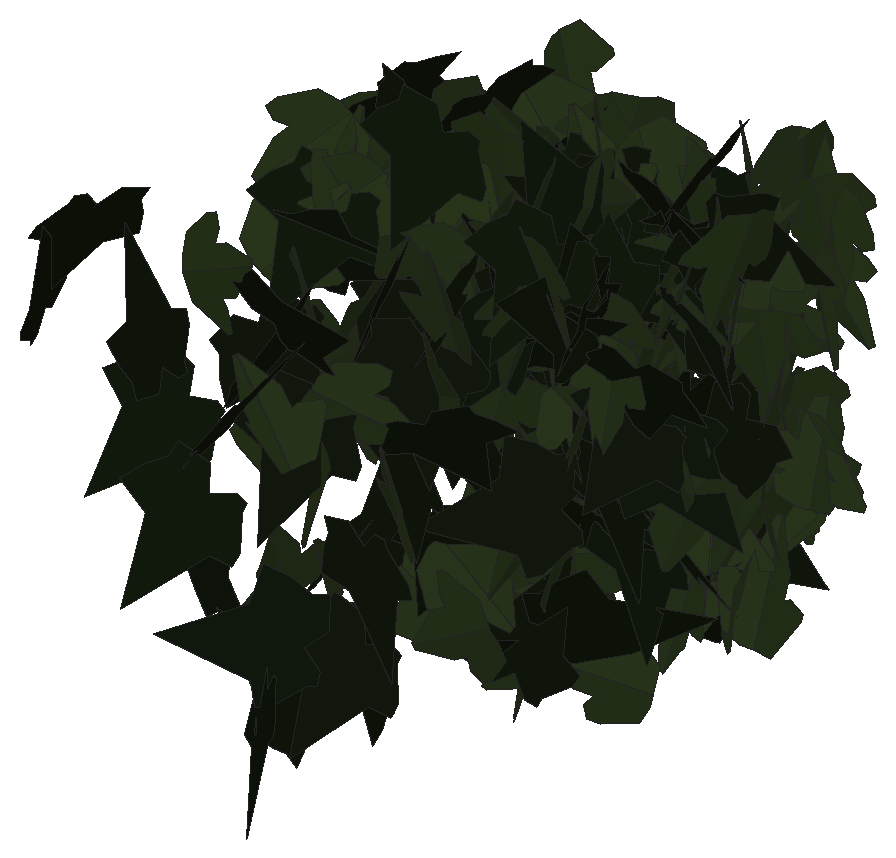
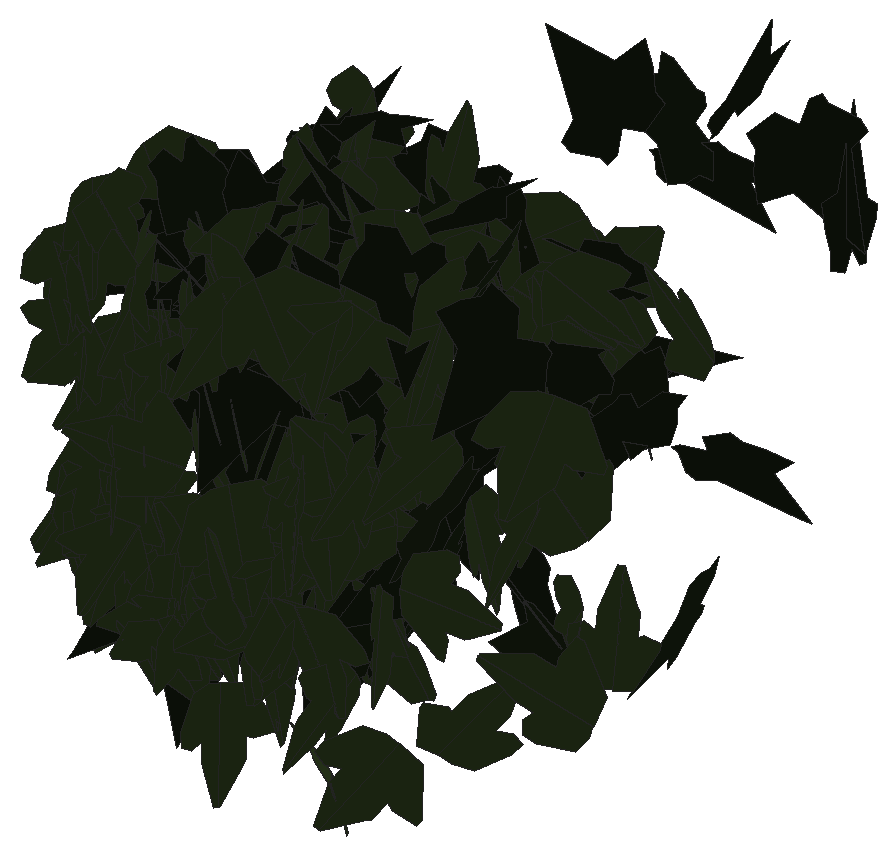
# SketchUp Ruby script. Lengths in inches.
U = 1.inch
M = Sketchup.active_model
def pt(a) = Geom::Point3d.new(a.map { |v| v * U })
def face(e, loops, mat)
  f = e.add_face(loops[0].map { |a| pt(a) })
  loops[1..].each { |l| e.add_face(l.map { |a| pt(a) }).erase! }
  f.material = f.back_material = mat if mat
  f
end
# faces: each face lists its corners as indices into pts; further lists are holes
def faces(e, pts, list, mat = nil) = list.each { |f| face(e, (f[0].is_a?(Array) ? f : [f]).map { |l| l.map { |i| pts[i] } }, mat) }
# xy, xz, yz: faces in a plane at the given z, y or x. An outline is a flat list of corners, or four numbers for a rectangle; further outlines are holes
def ring(l) = l.size == 4 ? [[l[0], l[1]], [l[2], l[1]], [l[2], l[3]], [l[0], l[3]]] : l.each_slice(2).to_a
def flat(e, list, mat, &to3) = list.each { |f| face(e, (f[0].is_a?(Array) ? f : [f]).map { |l| ring(l).map { |u, v| to3.(u, v) } }, mat) }
def xy(e, z, list, mat = nil) = flat(e, list, mat) { |x, y| [x, y, z] }
def xz(e, y, list, mat = nil) = flat(e, list, mat) { |x, z| [x, y, z] }
def yz(e, x, list, mat = nil) = flat(e, list, mat) { |y, z| [x, y, z] }
def lines(e, pts, list) = list.each { |a, b| e.add_line(pt(pts[a]), pt(pts[b])) }
# prism: a flat outline (further loops are holes) pulled along v
def prism(e, loops, v, mat = nil)
  f = face(e, loops, mat); d = Geom::Vector3d.new(v.map { |x| x * U })
  f.pushpull(f.normal.samedirection?(d) ? d.length : -d.length)
end
def box(e, o, s, mat = nil) = prism(e, [[o, [o[0] + s[0], o[1], o[2]], [o[0] + s[0], o[1] + s[1], o[2]], [o[0], o[1] + s[1], o[2]]]], [0, 0, s[2]], mat)
def at(x, y, z, deg = 0) = Geom::Transformation.translation(pt([x, y, z])) * Geom::Transformation.rotation(ORIGIN, Z_AXIS, deg.degrees)
def axes(o, x, y, z) = Geom::Transformation.new([*x, 0, *y, 0, *z, 0, *pt(o).to_a, 1])
def part(name) = M.definitions.add(name)
# library, detail: a bought-in or finely detailed component or shape, given as its bounding box
def library(name, o, s) = part(name).tap { |d| box(d.entities, o, s) }
def detail(e, o, s) = box(e.add_group.entities, o, s)
def put(e, d, t, mat = nil) = e.add_instance(d, t).tap { |i| i.material = mat if mat }
def group(e, t, mat = nil) = e.add_group.tap { |g| g.transformation = t; g.material = mat if mat }.entities
root = M.entities
M.materials.add("efeu1").color = [18, 25, 13]
M.materials.add("efeu2").color = [43, 57, 29]
c1 = part("ivyleaf_10")
p = [[0,0.5,-0.03],[-0.0625,2.02,-0.43],[-0.19,2.01,-0.46],[-0.54,1.05,-0.29],[-0.52,0.625,-0.18],[-0.83,0.76,-0.28],
  [-1.16,0.64,-0.33],[-1.15,0.33,-0.24],[-0.77,-0.39,0.02],[-0.3,-0.51,0.16],[0.04,-0.48,0.23],[-0.02,2.01,-0.4375],
  [-0.06,2.01,-0.43],[0.04,-0.49,0.23],[0.67,-0.49,0.14],[1.38,0.36,-0.2],[1.375,0.51,-0.24],[0.81,0.65,-0.19],
  [0.62,0.59,-0.15],[0.6,1.09,-0.28],[0.5,1.23,-0.31]]
faces(c1.entities,p,[[0,1,2,3,4,5,6,7,8,9,10],[11,12,0,13,14,15,16,17,18,19,20]],"efeu2")
c2 = part("ivyleaf_9")
p = [[1.54,2.16,1.25],[1.36,2.04,1.19],[-0.21,0.99,0.68],[-0.71,1.11,0.82],[-0.85,0.86,0.67],[-0.8,0.17,0.21],
  [-0.9,-0.01,0.1],[-0.67,-0.16,-0.02],[-0.08,-0.08,-0.05],[-0.03,-0.6,-0.4],[0.65,-0.88,-0.66],[0.83,-0.6,-0.49],
  [1.29,-0.42,-0.43],[1.8125,-0.07,-0.26],[1.21,0.44,0.15]]
faces(c2.entities,p,[[0,1,2,3,4,5,6,7,8,9,10,11,12,13,14]],"efeu1")
put(root,c1,axes([4.1875,224.93,203.2],[-0.1697,-0.07325,0.46458],[0.41933,0.2001,0.18472],[-0.21299,0.45232,-0.00648]))
put(root,c2,axes([4.59,220.26,206.02],[0.03494,0.24772,0.37035],[-0.11703,-0.34116,0.25706],[0.45365,-0.10709,0.03779]))
put(root,c1,axes([4.64,224.79,206.06],[-0.40343,-0.25391,-0.15091],[0.12885,0.07858,-0.47668],[0.26579,-0.4235,0.00203]))
put(root,c2,axes([4.91,221.93,204.38],[-0.43733,-0.15279,0.04548],[-0.04405,-0.01579,-0.45011],[0.16589,-0.40698,0.00039]))
put(root,c2,axes([5.05,220.43,207.12],[-0.05074,0.32429,-0.29754],[0.02517,-0.28547,-0.3405],[-0.46637,-0.05069,0.01399]))
put(root,c1,axes([5.375,223.53,206.75],[0.32878,0.07304,-0.3141],[-0.31526,-0.07769,-0.32554],[-0.11502,0.42173,-0.00557]))
put(root,c2,axes([5.04,222.01,202.73],[0.33996,-0.26991,-0.13674],[-0.10665,0.08682,-0.43124],[0.30621,0.3299,0.00162]))
put(root,c1,axes([4.91,222.18,205.66],[0.17929,-0.09629,-0.40599],[0.35577,-0.20958,0.19946],[-0.24898,-0.36882,-0.00735]))
put(root,c2,axes([5.21,224.53,206.61],[0.21832,0.33606,0.19573],[0.10391,0.16176,-0.40786],[-0.4028,0.22388,0.00088]))
put(root,c1,axes([5.71,225.24,204.04],[0.01886,0.02284,-0.45141],[-0.45168,0.11918,-0.01097],[0.12784,0.41773,0.02782]))
put(root,c2,axes([5.29,222.61,204.98],[0.08106,-0.27792,-0.33917],[-0.05368,0.3232,-0.29834],[0.45963,0.08676,0.02497]))
put(root,c1,axes([5.51,222.69,202.25],[-0.12317,-0.38419,-0.17594],[-0.02837,-0.16843,0.41622],[-0.45248,0.11514,0.0218]))
put(root,c1,axes([5.39,222.75,205.75],[0.27183,0.16125,-0.32867],[0.29159,0.16433,0.31083],[0.24859,-0.36908,-0.0052]))
put(root,c1,axes([5.71,223.23,206.21],[0.01419,0.31497,-0.31174],[0.01599,0.29939,0.32785],[0.46931,-0.01972,-0.00174]))
put(root,c2,axes([5.73,223.18,206.26],[-0.31837,-0.3187,0.02862],[-0.02124,-0.01929,-0.45149],[0.34482,-0.29544,-0.00139]))
put(root,c1,axes([5.59,223.17,203.97],[-0.15528,-0.36601,0.19342],[0.07202,0.17362,0.40897],[-0.43751,0.15849,-0.00133]))
put(root,c2,axes([5.71,223.18,202.38],[-0.22203,0.36028,-0.13624],[-0.07015,0.11376,0.4314],[0.40804,0.2156,0.00003]))
put(root,c2,axes([5.54,222.15,204.72],[0.09632,0.39174,0.17344],[-0.04238,-0.16211,0.41783],[0.45786,-0.09741,0.00218]))
put(root,c1,axes([5.89,223.38,206.35],[0.26009,0.1336,-0.35019],[-0.32984,-0.14257,-0.286],[-0.21041,0.38865,0.01546]))
put(root,c1,axes([5.77,222.7,205.28],[-0.35795,0.25236,0.13029],[0.09959,-0.08561,0.43306],[0.28752,0.34382,0.0122]))
put(root,c1,axes([5.85,223.49,204.02],[-0.06806,0.27457,0.34471],[-0.11059,0.31581,-0.29232],[-0.4515,-0.11874,0.01964]))
put(root,c1,axes([5.75,225.01,205.41],[0.04742,0.23194,0.37999],[0.05868,0.36139,-0.24538],[-0.4637,0.06945,0.00781]))
put(root,c2,axes([5.48,223.01,205.72],[0.29751,-0.01523,0.34976],[0.36233,-0.02377,-0.28691],[0.03028,0.43408,-0.00344]))
put(root,c1,axes([5.85,223.35,204.84],[0.08243,-0.36347,0.23552],[-0.01128,0.22839,0.38488],[-0.46237,-0.07037,0.03259]))
put(root,c1,axes([6.08,224.6875,206.58],[0.04798,0.09131,-0.48924],[-0.18918,-0.45127,-0.10278],[-0.46034,0.19497,-0.00875]))
put(root,c1,axes([6.05,224.69,206.42],[-0.44092,0.23576,-0.00349],[0.00297,-0.00185,-0.49999],[-0.23576,-0.44093,0.00023]))
put(root,c1,axes([5.91,225.62,202.35],[-0.365,-0.11682,-0.25762],[0.25231,0.08236,-0.37188],[0.15436,-0.41085,-0.0013]))
put(root,c1,axes([5.95,222.74,202.62],[-0.24505,0.2853,-0.24686],[0.15233,-0.19105,-0.37904],[-0.37075,-0.26707,0.00743]))
put(root,c2,axes([5.875,224.19,206.8],[0.11049,-0.37667,0.19972],[0.05839,-0.18431,-0.40591],[0.45287,0.11566,0.0036]))
put(root,c1,axes([6.16,223.84,204.05],[0.11861,-0.42089,0.00439],[0.00599,-0.00292,-0.45235],[0.45454,0.10986,0.00482]))
put(root,c2,axes([6.04,223.84,205.23],[0.01774,-0.29834,-0.32879],[-0.02163,0.31552,-0.31073],[0.46897,0.02584,-0.00189]))
put(root,c1,axes([6.3,224.01,201.72],[0.18967,0.31034,0.25911],[-0.13634,-0.21482,0.37083],[0.40762,-0.21625,0.00347]))
put(root,c1,axes([6.21,224.6,205.5],[-0.08774,-0.27767,-0.33784],[0.12661,0.30349,-0.30029],[0.44383,-0.14147,0.01888]))
put(root,c1,axes([6.28,225.4,205.21],[0.02776,-0.11632,-0.48549],[0.02716,0.48587,-0.11486],[0.49849,-0.01999,0.0333]))
put(root,c2,axes([6.41,222.98,202.81],[-0.3971,0.21835,-0.08288],[-0.08135,0.02916,0.44453],[0.23749,0.37509,0.01369]))
put(root,c2,axes([6.45,224.51,207.04],[0.05714,0.43158,-0.01349],[-0.00179,-0.01287,-0.4522],[-0.46631,0.05293,0.00008]))
put(root,c1,axes([6.34,225.85,206.84],[-0.01928,0.43461,-0.00484],[0.00288,-0.00455,-0.45237],[-0.4694,-0.01787,-0.00257]))
put(root,c2,axes([6.11,224.52,204.37],[0.21804,-0.41741,0.16801],[0.09712,-0.13864,-0.47048],[0.43935,0.2378,0.02062]))
put(root,c2,axes([6.09,224.21,206.42],[0.28246,-0.36735,0.18779],[0.11329,-0.14977,-0.46339],[0.39671,0.30433,-0.00137]))
put(root,c2,axes([6.3125,224.04,203.78],[0.32495,-0.22821,-0.22454],[-0.18254,0.13441,-0.39272],[0.286,0.34508,0.00447]))
put(root,c2,axes([6.57,219.5,206.44],[-0.12179,-0.33455,0.26431],[0.08473,0.24174,0.36715],[-0.44576,0.13736,-0.00242]))
put(root,c1,axes([6.63,224.68,203.27],[0.06532,-0.31686,-0.3035],[-0.05497,0.28737,-0.33547],[0.46198,0.07899,0.00299]))
put(root,c1,axes([6.75,225.37,201.76],[0.28586,-0.01067,0.35884],[-0.30725,0.23953,0.23467],[-0.21117,-0.36295,0.14432]))
put(root,c1,axes([6.65,223.71,206.62],[0.30392,0.25824,-0.21653],[-0.17165,-0.13468,-0.39715],[-0.31446,0.3231,0.00751]))
put(root,c1,axes([6.95,224.8,206.32],[-0.32488,0.05136,-0.32239],[-0.3354,0.01678,0.3163],[0.05169,0.43163,0.02607]))
put(root,c1,axes([6.45,225.2,206.56],[0.33672,0.25277,0.26969],[0.21818,0.15857,-0.42102],[-0.29836,0.40121,-0.00351]))
put(root,c1,axes([6.77,224.46,206.58],[-0.36671,-0.27159,0.01364],[-0.01095,-0.00833,-0.45219],[0.29345,-0.3397,0.00018]))
put(root,c1,axes([6.76,224.07,205.87],[-0.10194,-0.42462,0.00382],[-0.0007,-0.00362,-0.45238],[0.45861,-0.09439,0.00016]))
put(root,c2,axes([6.65,223.58,207.07],[-0.18972,-0.37844,0.12799],[0.01636,-0.14079,-0.42776],[0.42948,-0.16182,0.07283]))
put(root,c2,axes([6.4375,224.2,203.67],[0.45219,-0.10966,0.04531],[0.0455,-0.0111,-0.45013],[0.11904,0.42081,-0.00006]))
put(root,c1,axes([6.49,224.41,202.5],[0.36899,-0.14762,-0.23419],[0.22216,-0.09164,0.38706],[-0.18763,-0.39879,-0.00225]))
put(root,c1,axes([6.74,224.65,206.29],[-0.3796,-0.23626,-0.1033],[0.08975,0.05442,-0.44045],[0.26184,-0.36117,0.00121]))
put(root,c1,axes([6.92,225.6875,204.99],[-0.35044,0.24683,0.25743],[-0.22486,0.12722,-0.42808],[-0.27682,-0.4158,0.02184]))
put(root,c2,axes([6.86,224.59,206.06],[0.03769,0.43317,0.01992],[0.01042,0.01844,-0.45188],[-0.46817,0.03528,-0.00846]))
put(root,c1,axes([6.74,225.22,202.62],[-0.0201,0.24666,0.37214],[-0.05921,0.35396,-0.25672],[-0.46562,-0.05566,0.01658]))
put(root,c1,axes([6.79,224.74,205.96],[0.19796,0.35466,-0.17965],[-0.11675,-0.13803,-0.41403],[-0.40975,0.21068,0.03117]))
put(root,c1,axes([6.6875,224.875,205.64],[-0.34617,-0.21219,-0.21177],[0.20034,0.08785,-0.39887],[0.24647,-0.36943,0.02679]))
put(root,c1,axes([6.6875,225.25,205.1],[0.17132,0.27764,-0.30672],[0.15529,0.2575,0.33254],[0.40896,-0.21409,0.00222]))
put(root,c1,axes([6.9,225.24,204.6],[-0.36722,-0.26745,0.04743],[-0.04215,-0.02416,-0.44987],[0.28997,-0.34221,-0.00531]))
put(root,c2,axes([7.1,224.42,204.9],[-0.28827,-0.08559,0.34595],[-0.34028,-0.10674,-0.29149],[0.14771,-0.41292,0.00364]))
put(root,c1,axes([6.97,220.81,205.1],[0.37699,0.06883,0.2603],[-0.26494,-0.04966,0.37001],[0.09165,-0.42664,-0.00108]))
put(root,c1,axes([6.71,225.3,204.78],[0.40688,0.17958,-0.12757],[0.1197,0.05255,0.43404],[0.20208,-0.3927,-0.00025]))
put(root,c1,axes([6.53,225.01,204.43],[-0.02062,-0.00386,-0.45195],[0.46593,0.05222,-0.0202],[0.05653,-0.43184,0.0016]))
put(root,c1,axes([6.89,225.49,203.4],[0.49225,-0.03479,-0.08051],[-0.08032,0.00552,-0.49348],[0.03523,0.49876,-0.00016]))
put(root,c2,axes([7.18,221.91,202.37],[0.01916,0.01196,-0.45185],[-0.46822,-0.03043,-0.01928],[-0.03338,0.43377,0.01111]))
put(root,c1,axes([7.04,224.07,206.87],[-0.4832,-0.0062,0.12836],[-0.12806,-0.01896,-0.48295],[0.01085,-0.4996,0.01674]))
put(root,c1,axes([7.1,224.8125,204.15],[-0.14457,-0.02266,0.4298],[-0.16943,-0.39916,-0.07561],[0.41365,-0.17142,0.11925]))
put(root,c2,axes([6.75,224.66,206.04],[0.19302,0.39535,0.03259],[-0.02879,-0.02232,0.45095],[0.42735,-0.18007,0.01566]))
put(root,c2,axes([6.75,224.58,205.84],[0.30492,0.04251,0.34132],[0.26166,0.2673,-0.25277],[-0.24345,0.34054,0.15581]))
put(root,c1,axes([7.07,225.18,204.66],[0.27383,0.28604,-0.21596],[-0.16674,-0.14026,-0.397],[-0.3434,0.2962,0.02056]))
put(root,c2,axes([7.0625,222.37,206.32],[-0.26031,0.19627,-0.31649],[0.25558,-0.19134,-0.32326],[-0.29603,-0.33778,-0.00079]))
put(root,c1,axes([6.95,224.34,206.0625],[0.03067,-0.14695,-0.42478],[0.06462,-0.40408,0.15552],[-0.46432,-0.06595,-0.00642]))
put(root,c1,axes([7.12,225.27,204.12],[0.13945,0.24481,-0.34902],[-0.15471,-0.30363,-0.28767],[-0.42111,0.19262,-0.00989]))
put(root,c2,axes([6.75,224.11,205.75],[0.20544,-0.18803,-0.35677],[0.40603,-0.0176,0.22684],[-0.11681,-0.39187,0.16101]))
put(root,c2,axes([7.16,221.07,205.34],[-0.39959,-0.20611,-0.10319],[0.0935,0.04848,-0.44047],[0.22868,-0.37999,-0.00022]))
put(root,c1,axes([7.02,222.82,206.36],[-0.39804,-0.11368,-0.20922],[0.2037,0.07079,-0.40096],[0.14417,-0.41387,-0.01112]))
put(root,c2,axes([6.72,224.38,205.27],[0.33615,0.08318,-0.36067],[0.34408,0.10935,0.3459],[0.13642,-0.48075,0.01628]))
put(root,c1,axes([7.14,223.74,205.23],[-0.07646,-0.39956,-0.16301],[0.10948,0.1388,-0.41559],[0.45042,-0.10156,0.07335]))
put(root,c1,axes([7.08,224.91,204.2],[-0.27523,-0.28491,-0.21592],[0.21066,0.09944,-0.39092],[0.31715,-0.31331,0.07228]))
put(root,c2,axes([7.02,224.38,205.26],[0.14069,-0.4475,-0.17306],[-0.04406,0.16753,-0.46903],[0.47777,0.14723,0.0077]))
put(root,c1,axes([7.15,225.32,203.26],[-0.06355,0.41424,-0.12379],[0.02021,-0.11757,-0.43513],[-0.46504,-0.06171,-0.00199]))
put(root,c1,axes([7.36,223.66,204.5625],[-0.34583,-0.25925,0.14514],[-0.10732,-0.09892,-0.42825],[0.29932,-0.33501,0.01414]))
put(root,c1,axes([7.37,225.54,206.68],[-0.21891,-0.41701,0.16787],[-0.05523,-0.16035,-0.47036],[0.44613,-0.22448,0.02415]))
put(root,c2,axes([7.39,219.14,205.43],[-0.42486,-0.18545,-0.00949],[0.00857,0.00458,-0.4523],[0.20034,-0.39346,-0.00079]))
put(root,c2,axes([7.14,224.39,204.49],[-0.03088,-0.37745,-0.22291],[0.04429,0.21149,-0.39303],[0.46669,-0.04504,0.02255]))
put(root,c1,axes([7.27,225.47,203.29],[-0.35355,-0.27119,-0.09599],[0.1514,-0.02942,-0.42717],[0.26981,-0.33885,0.11391]))
put(root,c2,axes([7.66,223.83,203.21],[-0.42781,-0.00958,0.18668],[-0.19381,-0.00408,-0.41209],[0.01124,-0.43488,-0.00025]))
put(root,c2,axes([7.29,219.28,205.92],[-0.09415,0.40895,-0.12474],[-0.02748,0.11721,0.43486],[0.45945,0.09082,0.00045]))
put(root,c1,axes([7.17,224.49,204.6],[0.29831,-0.21627,0.33799],[0.27285,-0.19947,-0.36846],[0.29421,0.40428,-0.00099]))
put(root,c2,axes([7.51,220.33,202.65],[0.00879,-0.42348,0.10308],[0.0016,0.09916,0.44049],[-0.46972,-0.00758,0.00343]))
put(root,c1,axes([7.34,225.39,203.78],[0.24286,0.36958,-0.04731],[-0.04172,-0.0297,-0.44955],[-0.39999,0.22749,0.01817]))
put(root,c2,axes([7.09,224.6,202.4],[0.1331,-0.26789,0.40065],[0.15376,-0.37033,-0.29869],[0.45677,0.20272,-0.0162]))
put(root,c1,axes([7.47,220.75,204.91],[0.24236,-0.35034,-0.13208],[-0.06309,0.11334,-0.43253],[0.39748,0.23161,0.01188]))
put(root,c2,axes([7.76,220.0625,203.56],[-0.23864,-0.04809,0.38646],[-0.39428,-0.06951,-0.23512],[0.09112,-0.42671,-0.00525]))
put(root,c1,axes([7.68,225.17,203.84],[-0.1435,-0.09106,0.47023],[-0.23369,-0.41518,-0.15171],[0.41809,-0.26331,0.0766]))
put(root,c2,axes([7.11,220.58,206.55],[0.04935,-0.16782,0.41466],[0.34583,-0.25645,-0.15042],[0.31413,0.3087,0.10046]))
put(root,c1,axes([7.46,224.32,203.82],[-0.16746,-0.39234,-0.11031],[0.07573,0.086,-0.43743],[0.43236,-0.16702,0.0339]))
put(root,c1,axes([7.54,225.23,202.8125],[0.04902,-0.43069,-0.04247],[-0.00393,0.04068,-0.4504],[0.46722,0.04553,0.00067]))
put(root,c1,axes([7.66,225.66,204.41],[-0.3214,-0.37286,0.08762],[-0.05151,-0.07127,-0.49221],[0.37954,-0.32541,0.0074]))
put(root,c1,axes([7.63,225.86,202.42],[-0.13847,-0.40686,-0.08857],[0.01084,0.08607,-0.44333],[0.4488,-0.12761,-0.01662]))
put(root,c1,axes([7.33,221.14,205.59],[-0.21204,-0.09863,-0.39045],[0.38042,0.13152,-0.22751],[0.17616,-0.40274,0.02133]))
put(root,c2,axes([7.75,222.47,206.22],[-0.34524,0.24405,-0.1724],[0.12809,-0.11749,-0.41776],[-0.29175,-0.34038,0.02059]))
put(root,c2,axes([7.75,222.59,203.74],[0.1046,0.30543,-0.30598],[-0.09001,-0.28219,-0.3332],[-0.44908,0.1277,-0.00448]))
put(root,c1,axes([7.54,224.45,203.72],[-0.41875,-0.23529,0.13887],[0.1232,0.06423,0.48031],[-0.24386,0.43648,0.00418]))
put(root,c1,axes([7.57,225.75,203.47],[0.16823,-0.40079,0.06846],[-0.02313,0.0623,0.44718],[-0.43804,-0.15721,0.00268]))
put(root,c2,axes([7.43,222.09,204.62],[0.093,-0.36424,0.23054],[0.06071,-0.21448,-0.38922],[0.45648,0.10273,0.0048]))
put(root,c2,axes([7.5625,222.23,205.72],[-0.25521,-0.29402,-0.22531],[0.15826,0.16003,-0.3921],[0.36129,-0.27779,0.0126]))
put(root,c1,axes([7.59,224.85,207.01],[-0.13893,0.38783,-0.15519],[0.06137,-0.13832,-0.42483],[-0.44457,-0.1403,-0.01015]))
put(root,c2,axes([7.74,223.79,202.68],[0.16494,0.39805,0.08979],[0.0289,0.08221,-0.44338],[-0.43894,0.15499,0.00455]))
put(root,c1,axes([7.73,223.76,206.88],[0.25356,-0.43088,0.00715],[0.00363,-0.00617,-0.49995],[0.43092,0.25359,0]))
put(root,c2,axes([7.46,223.26,204.125],[0.27225,-0.34537,0.0832],[0.0418,-0.07076,-0.44456],[0.38058,0.25483,-0.01069]))
put(root,c1,axes([7.49,225.61,203.39],[-0.30023,-0.0203,-0.34733],[0.36028,0.01658,-0.28983],[0.02779,-0.43421,0.00517]))
put(root,c2,axes([7.79,220.98,203.15],[-0.20705,-0.36079,0.15531],[-0.08144,-0.12902,-0.42487],[0.41377,-0.20594,-0.00591]))
put(root,c1,axes([7.71,224.46,205.71],[0.29254,-0.33758,0.04519],[-0.0124,0.04644,0.44966],[-0.36739,-0.27038,0.02081]))
put(root,c2,axes([8.02,224.56,206.08],[0.01218,0.00011,0.45225],[-0.44752,-0.13194,0.01121],[0.14245,-0.41451,-0.00345]))
put(root,c1,axes([7.9,224.44,206.46],[0.42066,0.08893,0.17896],[-0.18112,-0.03855,0.4155],[0.10467,-0.42407,-0.00024]))
put(root,c1,axes([7.97,223.54,201.97],[-0.28957,-0.18731,-0.29827],[-0.21944,-0.20625,0.33764],[-0.29784,0.33407,0.04122]))
put(root,c2,axes([8,224.27,206.26],[-0.45016,0.09424,-0.08457],[0.08432,-0.02338,-0.44439],[-0.10469,-0.42403,0.00571]))
put(root,c1,axes([7.66,222.54,203.39],[0.18535,0.30899,0.26371],[0.12534,0.22555,-0.36753],[-0.41309,0.20708,0.00681]))
put(root,c1,axes([7.92,221.43,204.26],[-0.35373,0.28626,-0.00213],[-0.00663,-0.00391,0.45234],[0.3091,0.32752,0.00726]))
put(root,c2,axes([7.76,219.59,203.21],[-0.25207,0.0761,-0.37347],[0.37458,-0.09367,-0.25508],[-0.12985,-0.41792,-0.01083]))
put(root,c1,axes([7.85,224.98,204.5],[-0.17575,-0.40161,-0.03965],[-0.01572,-0.03524,0.45066],[-0.4354,0.16338,-0.00027]))
put(root,c2,axes([7.67,221.17,204.05],[0.12828,-0.41288,0.07093],[0.02783,-0.06354,-0.44674],[0.45109,0.12133,0.00739]))
put(root,c1,axes([8,222.01,206.12],[-0.44166,0.14344,-0.03907],[-0.03888,0.01085,0.45071],[0.15535,0.41053,0.00174]))
put(root,c1,axes([7.97,225.17,203.78],[0.07163,-0.28898,-0.33104],[0.00465,0.3225,-0.30357],[0.46428,0.04135,0.05411]))
put(root,c1,axes([8.17,223.9,205.66],[-0.07259,-0.10732,0.43281],[-0.21378,-0.36615,-0.13144],[0.412,-0.2089,0.00805]))
put(root,c1,axes([8.07,223.79,202.83],[-0.07954,-0.32659,0.28885],[-0.06148,-0.27187,-0.34816],[0.45892,-0.09303,0.00342]))
put(root,c1,axes([7.81,225.02,204.44],[-0.06179,0.00803,0.44839],[0.28686,-0.34197,0.04328],[0.36688,0.26873,0.04167]))
put(root,c2,axes([8.34,223.42,206.71],[-0.41207,0.04281,-0.27994],[-0.27955,0.01765,0.41418],[0.04535,0.49785,0.00939]))
put(root,c1,axes([7.74,223.43,202.67],[-0.20154,-0.16459,0.42696],[0.32579,0.27598,0.26018],[-0.32131,0.38307,-0.004]))
put(root,c1,axes([7.875,223.54,202.2],[0.11876,-0.19138,0.38984],[0.22211,-0.31359,-0.22925],[0.39658,0.23294,0.01165]))
put(root,c2,axes([8,224.49,206.72],[-0.29786,-0.33284,-0.05077],[0.07713,0.00375,-0.44624],[0.35503,-0.28006,0.05436]))
put(root,c2,axes([8.16,224.84,205.26],[0.22583,0.32621,-0.20562],[-0.17776,-0.12624,-0.39765],[-0.37164,0.25861,0.06526]))
put(root,c2,axes([8.21,222.6875,205.97],[-0.45291,0.06041,-0.1025],[0.1037,-0.0245,-0.4405],[-0.06952,-0.43009,0.01069]))
put(root,c2,axes([8.04,224.85,205.49],[0.26324,0.35957,0.02385],[0.01594,0.0177,-0.45176],[-0.3888,0.24418,-0.00238]))
put(root,c1,axes([8.03,224.25,202.79],[-0.26889,0.3475,-0.0837],[0.04542,-0.06887,-0.44455],[-0.38255,-0.25243,0.00605]))
put(root,c1,axes([8.15,224.7,206.08],[-0.2371,-0.37449,-0.02912],[0.0092,0.02746,-0.45141],[0.40547,-0.21961,-0.00678]))
put(root,c1,axes([8.01,225.17,206.26],[-0.14337,-0.34624,-0.331],[0.20114,0.27006,-0.36961],[0.43473,-0.23914,0.06185]))
put(root,c2,axes([7.87,223.28,201.99],[0.28138,0.34815,0.012],[-0.00913,-0.00809,0.45224],[0.3761,-0.26067,0.002]))
put(root,c1,axes([8.45,221.87,203.17],[-0.22839,-0.00117,0.39534],[-0.40754,-0.05194,-0.21849],[0.04963,-0.43189,0.02521]))
put(root,c2,axes([7.9,224.16,206.59],[0.13149,-0.04528,-0.48027],[0.06783,0.49458,-0.02806],[0.47761,-0.05778,0.1362]))
put(root,c1,axes([8.15,224.92,204.99],[0.21432,-0.3849,0.04287],[0.03521,-0.02954,-0.45008],[0.41658,0.20052,0.01599]))
put(root,c1,axes([7.93,223.57,202.1],[-0.32706,-0.08759,0.31173],[0.32518,0.02885,0.32514],[-0.08946,0.42511,0.04216]))
put(root,c2,axes([8.07,222.9375,202.18],[-0.30044,0.10991,0.32848],[0.29183,-0.16818,0.30838],[0.21279,0.38582,0.04085]))
put(root,c1,axes([8.125,224.64,205.87],[0.41923,0.19568,-0.0166],[-0.01467,-0.00851,-0.45209],[-0.21153,0.38841,-0.00154]))
put(root,c1,axes([8.12,223.24,203.75],[0.04949,-0.22112,0.44571],[0.15438,-0.41898,-0.225],[0.47299,0.15989,0.0268]))
put(root,c1,axes([7.96,221.92,205.47],[-0.20854,0.10829,0.38943],[0.36032,-0.17018,0.23011],[0.2177,0.3854,-0.00781]))
put(root,c1,axes([8.35,224.89,203.14],[0.10969,0.2687,0.33973],[-0.16312,-0.29077,0.29757],[0.4267,-0.18022,0.02642]))
put(root,c1,axes([8.28,224.78,205.7],[-0.08884,-0.42106,0.07475],[-0.03113,-0.06755,-0.4459],[0.46027,-0.08584,-0.01573]))
put(root,c1,axes([8.27,225.68,202.99],[-0.04487,0.36422,-0.24355],[-0.13072,-0.23565,-0.35883],[-0.44901,0.03221,0.12881]))
put(root,c1,axes([8.17,224.75,206.93],[0.09806,0.42054,0.0668],[0.01484,0.06275,-0.44744],[-0.45921,0.09183,-0.0002]))
put(root,c1,axes([8.29,225.25,203.16],[0.09335,-0.48263,0.09139],[0.01322,-0.09053,-0.49156],[0.49103,0.09418,-0.00414]))
put(root,c1,axes([8.4,222.84,206.42],[-0.18845,-0.3965,-0.04116],[0.00772,0.04009,-0.45041],[0.43028,-0.17437,-0.00995]))
put(root,c1,axes([8.34,225.08,206.73],[0.44589,-0.13321,-0.03329],[-0.03144,0.01403,-0.45115],[0.14459,0.41386,0.00458]))
put(root,c1,axes([8.23,223.71,204.76],[0.27794,0.3356,0.1059],[0.0664,0.08117,-0.43983],[-0.3729,0.26459,0.00062]))
put(root,c1,axes([8.38,223.21,203.02],[0.13664,-0.34971,0.3302],[-0.12404,0.30603,0.37544],[-0.4647,-0.18452,-0.00313]))
put(root,c2,axes([8.58,223.75,204.48],[-0.29949,0.3343,-0.02483],[0.0219,-0.01419,-0.45167],[-0.3613,-0.27797,-0.0068]))
put(root,c2,axes([7.97,223.34,203.66],[0.26474,-0.08012,0.36433],[0.35753,-0.11462,-0.26818],[0.15098,0.41191,-0.00376]))
put(root,c1,axes([8.72,225.3,203.61],[0.02869,0.03233,-0.4503],[-0.46875,0.01378,-0.02662],[0.01276,0.43358,0.03443]))
put(root,c1,axes([8.42,225.06,204.8],[0.10653,-0.42009,0.05717],[-0.0033,-0.05715,-0.44847],[0.45755,0.0974,-0.01654]))
put(root,c1,axes([8.37,225.42,203.34],[-0.32465,-0.28609,-0.13566],[0.11949,0.07268,-0.43094],[0.31786,-0.31952,0.02344]))
put(root,c1,axes([8.4,225.69,202.875],[0.39457,0.20261,-0.12611],[-0.10624,-0.07248,-0.43419],[-0.23183,0.37805,-0.01566]))
put(root,c1,axes([8.36,224.34,206.01],[-0.33626,-0.25324,-0.17449],[0.14406,0.10189,-0.41737],[0.29477,-0.33869,0.00492]))
put(root,c1,axes([8.44,223.57,206.99],[-0.01701,-0.19245,-0.40539],[0.04094,0.38796,-0.2008],[0.4677,-0.04096,0.00283]))
put(root,c1,axes([8.41,225.05,205.23],[0.24554,-0.36636,0.05992],[0.04057,-0.04448,-0.44833],[0.39847,0.23028,0.00873]))
put(root,c1,axes([8.53,223.97,203.11],[0.02443,0.12584,0.43242],[-0.07121,-0.41053,0.13295],[0.46373,-0.06967,-0.00236]))
put(root,c2,axes([8.76,223.54,204.18],[0.08282,0.05507,0.44162],[-0.38612,0.24563,0.03402],[-0.25448,-0.35477,0.0921]))
put(root,c2,axes([8.6,223.51,205.95],[-0.37876,-0.18149,0.18977],[0.17443,0.08491,0.41067],[-0.2164,0.3861,-0.00111]))
put(root,c2,axes([8.78,222.63,204.25],[-0.29155,-0.10171,0.3386],[-0.33065,-0.11082,-0.30001],[0.16242,-0.40817,-0.00293]))
put(root,c1,axes([8.5625,223.24,205.6875],[-0.3201,-0.31626,-0.03838],[0.03986,0.01596,-0.45046],[0.34156,-0.29825,0.0166]))
put(root,c2,axes([8.88,223.625,204.5],[-0.38555,0.18715,0.17012],[-0.16817,0.05474,-0.41857],[-0.20924,-0.38885,0.02295]))
put(root,c2,axes([8.52,221.08,205.72],[0.33736,0.30194,-0.02281],[-0.01707,-0.01521,-0.45182],[-0.32651,0.31277,0.00005]))
put(root,c1,axes([8.8125,223.24,205.86],[-0.36506,0.10953,0.26097],[-0.28026,-0.00102,-0.36308],[-0.0943,-0.42098,0.06878]))
put(root,c1,axes([8.47,225.61,203.03],[0.33083,0.30502,0.05046],[0.0379,0.03351,-0.44958],[-0.3314,0.30832,-0.00105]))
put(root,c1,axes([8.32,225.02,206.08],[0.29427,-0.21472,-0.3425],[0.26678,-0.21512,0.36407],[-0.3037,-0.39701,-0.01204]))
put(root,c2,axes([8.81,224.26,204.17],[-0.46974,-0.00037,0.00745],[-0.00773,-0.00406,-0.45232],[0.00047,-0.43498,0.00422]))
put(root,c2,axes([8.39,224.79,205.72],[0.18209,-0.39451,-0.07468],[-0.00956,0.07421,-0.44567],[0.43297,0.16756,0.02156]))
put(root,c1,axes([8.64,224.95,206.06],[0.11858,-0.48571,-0.00485],[-0.00136,0.00466,-0.49998],[0.48573,0.11859,-0.00022]))
put(root,c2,axes([8.78,224.6875,206.36],[0.15055,0.32578,-0.2624],[-0.18935,-0.19415,-0.36145],[-0.40273,0.21307,0.07185]))
put(root,c1,axes([8.66,223.51,206],[-0.46626,0.05325,-0.00299],[0.00264,-0.00369,-0.45238],[-0.05753,-0.43171,0.0035]))
put(root,c1,axes([8.63,222.41,206.51],[0.05127,-0.41866,0.11246],[0.03835,-0.10464,-0.43756],[0.46542,0.05474,0.02366]))
put(root,c1,axes([8.92,223.56,202.01],[0.08139,0.06026,0.44113],[-0.37368,-0.24542,0.1002],[0.27286,-0.35407,0.00563]))
put(root,c2,axes([8.65,222.76,206.9375],[-0.31137,-0.32402,0.03478],[0.05042,-0.0853,-0.44095],[0.34817,-0.27742,0.09496]))
put(root,c1,axes([8.5,225,205.74],[0.08495,-0.1098,0.48034],[0.25785,-0.40545,-0.13828],[0.41988,0.27121,-0.01226]))
put(root,c1,axes([8.73,224.99,205.54],[0.01514,0.30909,-0.31799],[-0.16077,-0.28402,-0.3057],[-0.44118,0.1141,0.10048]))
put(root,c2,axes([8.52,224.79,206.39],[0.04851,-0.36473,-0.24207],[-0.01986,0.23219,-0.38208],[0.46687,0.04777,0.0089]))
put(root,c1,axes([8.75,224.81,206.07],[0.08734,-0.33221,-0.27969],[-0.05983,0.26325,-0.35552],[0.45772,0.0978,0.00689]))
put(root,c1,axes([8.78,225.47,203.21],[-0.16489,-0.38141,0.14868],[-0.05407,-0.13394,-0.42726],[0.43658,-0.16065,0.00324]))
put(root,c1,axes([8.57,225.45,203.68],[-0.3343,0.22012,-0.22052],[0.13696,-0.18208,-0.38912],[-0.30033,-0.32805,0.06801]))
put(root,c2,axes([9.01,224.9,206.36],[-0.39109,0.21654,0.1101],[-0.10811,0.0387,-0.43841],[-0.2368,-0.37529,0.01832]))
put(root,c2,axes([8.63,222.63,206.02],[0.31545,0.31129,0.08708],[0.061,0.06182,-0.44394],[-0.34276,0.29749,0.00113]))
put(root,c1,axes([8.65,225.09,205.41],[0.17415,0.32196,0.25382],[0.06315,0.24141,-0.37139],[-0.43174,0.16518,0.04806]))
put(root,c1,axes([8.79,223.07,205.2],[0.22735,-0.37953,-0.03069],[-0.00992,0.02865,-0.45132],[0.41101,0.21063,0.00608]))
put(root,c1,axes([8.7,222.46,207],[-0.35202,0.2639,-0.12012],[0.10762,-0.06036,-0.43587],[-0.29191,-0.34049,-0.01583]))
put(root,c2,axes([8.85,224.64,202.5],[0.15027,0.41191,-0.01472],[-0.0069,-0.01278,-0.45216],[-0.44507,0.13927,0.00204]))
put(root,c1,axes([8.84,224.87,205.62],[-0.08976,-0.4035,0.14523],[0.03347,-0.1476,-0.42434],[0.45993,-0.06801,0.05923]))
put(root,c2,axes([8.4375,224.46,206.61],[0.3019,-0.19916,0.27794],[0.23807,-0.15114,-0.35693],[0.26998,0.35598,0.00395]))
put(root,c1,axes([8.58,225.59,204.64],[-0.10865,-0.12766,0.41963],[0.27758,0.31107,0.169],[-0.36312,0.27598,0.00362]))
put(root,c2,axes([8.46,223.21,202.58],[0.19885,-0.0075,0.45869],[0.45851,0.01948,-0.19846],[-0.01489,0.49956,0.01462]))
put(root,c2,axes([8.59,224.84,205.52],[0.19983,-0.3551,0.17678],[0.09513,-0.14572,-0.4163],[0.4144,0.20469,0.01032]))
put(root,c2,axes([9.03,224.65,207.17],[-0.2323,0.33757,-0.17712],[0.08527,-0.15152,-0.41604],[-0.39934,-0.22872,0.0142]))
put(root,c2,axes([8.75,224.16,204.3125],[0.40696,-0.21425,-0.03797],[0.03329,-0.01965,0.4508],[-0.23235,-0.37807,-0.00192]))
put(root,c1,axes([9.1,225.29,206.3],[-0.21403,0.2546,-0.30344],[-0.18233,0.23817,0.33539],[0.37637,0.26016,-0.01008]))
put(root,c2,axes([9.06,222.64,206.26],[-0.11688,0.15052,-0.40926],[-0.30971,0.27134,0.18996],[0.33337,0.30486,0.03299]))
put(root,c2,axes([8.95,222.88,206.28],[-0.06141,-0.0367,0.49486],[-0.22876,-0.44039,-0.06105],[0.44034,-0.2339,0.03729]))
put(root,c1,axes([8.95,225.23,204.73],[0.14334,-0.38427,-0.16095],[0.01503,0.16655,-0.41768],[0.44715,0.11759,0.06563]))
put(root,c1,axes([9.07,225.45,205.875],[-0.002,-0.01185,-0.49986],[-0.09277,0.49119,-0.01127],[0.49132,0.09269,-0.00416]))
put(root,c1,axes([9.15,225.49,204.625],[-0.17298,0.24965,0.33092],[-0.25707,0.2185,-0.3029],[-0.35314,-0.28135,0.0584]))
put(root,c2,axes([8.82,225.05,203.11],[0.01588,-0.08936,-0.44249],[0.03795,0.42456,-0.09147],[0.468,-0.03139,0.02244]))
put(root,c2,axes([8.78,225.09,205.08],[0.18443,-0.4,-0.00813],[0.00112,0.00894,-0.4523],[0.43208,0.17072,0.00464]))
put(root,c1,axes([9.02,224.63,206.59],[0.346,-0.26885,-0.12441],[-0.0443,0.13431,-0.42818],[0.3147,0.3145,0.07651]))
put(root,c1,axes([8.93,224.73,203.09],[0.4149,0.20405,0.00198],[0.00177,0.00096,-0.4524],[-0.22038,0.38417,0.00008]))
put(root,c2,axes([8.84,223.83,203.46],[0.04584,-0.42242,0.09856],[0.02606,-0.09277,-0.44128],[0.46683,0.04666,0.01495]))
put(root,c1,axes([9.02,224.25,202.8],[0.41179,-0.20906,-0.0123],[-0.01042,0.007,-0.45223],[0.22591,0.38141,0.00156]))
put(root,c2,axes([8.8125,223.45,204.24],[0.13905,-0.39498,0.13415],[0.04633,-0.12168,-0.43204],[0.44635,0.13568,0.00305]))
put(root,c1,axes([9.06,225.09,205.46],[-0.45559,0.10002,-0.03709],[0.03503,-0.01775,-0.45076],[-0.10921,-0.42297,0.01014]))
put(root,c1,axes([9.05,224.96,206.05],[0.1904,-0.39512,0.04679],[0.09652,-0.00859,-0.44266],[0.4185,0.18175,0.08081]))
put(root,c2,axes([8.97,223.91,203.6],[0.42922,-0.09695,-0.15383],[-0.13916,0.09047,-0.42173],[0.13083,0.4143,0.05609]))
put(root,c1,axes([8.97,225.6,203.63],[0.20774,0.33945,0.20005],[0.10853,0.16413,-0.40572],[-0.40716,0.21694,-0.00607]))
put(root,c1,axes([9.15,225.63,203.6],[-0.46673,0.0311,-0.0402],[0.04014,-0.0216,-0.45019],[-0.0355,-0.43335,0.01956]))
put(root,c2,axes([9.45,224.57,204.58],[-0.03481,0.02461,-0.45043],[-0.24061,-0.37359,-0.00483],[-0.402,0.22148,0.0419]))
put(root,c1,axes([9.19,225.59,204],[-0.46491,-0.05327,-0.0342],[0.04139,-0.04353,-0.44836],[0.05346,-0.42953,0.04968]))
put(root,c2,axes([9.22,224.05,204.99],[-0.13286,0.14546,-0.40671],[0.23153,-0.32774,-0.19692],[-0.38659,-0.24627,0.02184]))
put(root,c1,axes([9.16,225.01,206.11],[0.45644,0.103,-0.00121],[-0.00059,-0.00268,-0.45239],[-0.11125,0.42262,-0.00258]))
put(root,c1,axes([9.18,224.86,205.93],[0.28761,-0.3339,0.08587],[0.08706,-0.04092,-0.44252],[0.36113,0.27579,0.03829]))
put(root,c1,axes([9.34,225.07,203.6],[-0.07954,-0.42322,0.25409],[-0.04024,-0.25095,-0.43059],[0.49199,-0.08895,0.00587]))
put(root,c1,axes([9.28,225.49,204.38],[-0.28215,-0.39608,-0.11622],[0.06845,0.09393,-0.4863],[0.40707,-0.29034,0.00122]))
put(root,c1,axes([9.46,224.95,203.54],[-0.15164,0.17254,0.38877],[-0.30299,0.24898,-0.2291],[-0.32545,-0.31219,0.03214]))
put(root,c2,axes([9.06,224.65,206.45],[0.02603,-0.00483,-0.45168],[0.10281,0.42445,0.00059],[0.45767,-0.09508,0.02556]))
put(root,c1,axes([9.36,224.98,205.38],[-0.42577,-0.18369,-0.00829],[0.00891,0.00117,-0.45232],[0.19837,-0.39431,0.00252]))
put(root,c1,axes([9.22,222.9,205.84],[0.4481,-0.11895,0.05631],[0.058,-0.00914,-0.44884],[0.12868,0.41832,0.00621]))
put(root,c1,axes([9.36,225.48,207.03],[0.08964,0.37947,-0.20364],[-0.14033,-0.16757,-0.39501],[-0.4393,0.13096,0.08464]))
put(root,c1,axes([9.33,225.61,203.68],[0.3616,0.25941,-0.1031],[-0.08887,-0.05564,-0.44045],[-0.28646,0.34472,0.0065]))
put(root,c1,axes([9.23,225.28,205.34],[-0.1514,-0.23191,-0.35389],[0.2291,0.26743,-0.28043],[0.38119,-0.25283,0.02799]))
put(root,c2,axes([9.32,223.33,205.04],[-0.21407,-0.32873,0.21281],[0.00202,-0.23069,-0.38354],[0.41819,-0.16717,0.11079]))
put(root,c1,axes([9.2,224.04,204.53],[-0.23463,0.20932,-0.32592],[0.23326,-0.22728,-0.31359],[-0.33355,-0.30619,0.00996]))
put(root,c1,axes([9.41,225.59,203.63],[0.43204,0.15432,-0.07628],[-0.10179,0.04355,-0.43933],[-0.15392,0.40437,0.07642]))
put(root,c1,axes([9.43,225.5,207.03],[-0.0414,-0.42875,-0.06518],[0.04961,0.05854,-0.44573],[0.46533,-0.04439,0.04173]))
put(root,c1,axes([9.5,225.63,206.57],[-0.35678,-0.27816,-0.05422],[0.04242,0.03429,-0.44914],[0.30269,-0.33268,-0.00097]))
put(root,c1,axes([9.52,224.6875,202.41],[0.0837,0.38328,-0.30999],[0.02064,0.31142,0.39063],[0.49251,-0.07819,0.03631]))
put(root,c1,axes([9.46,225,204.45],[0.21058,-0.43941,0.11213],[-0.04631,0.10215,0.48726],[-0.45112,-0.2156,0.00232]))
put(root,c1,axes([9.32,224.62,202.625],[0.12687,-0.31475,-0.28738],[0.15403,-0.23978,0.3471],[-0.42531,-0.18073,0.03998]))
put(root,c1,axes([9.26,223.73,204.36],[0.05955,-0.06094,-0.44425],[0.28625,-0.33504,0.08528],[-0.36773,-0.27067,-0.00555]))
put(root,c1,axes([9.56,225.46,203.59],[0.08218,0.41793,-0.26188],[0.03798,0.25934,0.42579],[0.49174,-0.08988,0.01088]))
put(root,c2,axes([9.65,222.75,205.98],[0.32183,0.18054,-0.27086],[-0.26669,-0.09179,-0.36],[-0.21451,0.38497,0.04119]))
put(root,c1,axes([9.7,223.58,204.32],[-0.27877,-0.32077,0.146],[-0.08321,-0.1181,-0.42797],[0.36889,-0.26905,0.01379]))
put(root,c2,axes([9.38,223.43,204.86],[0.09618,-0.29839,-0.31589],[0.02562,0.31331,-0.31287],[0.45914,0.04502,0.08363]))
put(root,c1,axes([9.58,225.81,206.39],[-0.42969,0.14949,-0.09635],[0.035,-0.1629,-0.41812],[-0.18669,-0.37462,0.14337]))
put(root,c1,axes([9.42,225.81,205.76],[-0.36705,0.04348,-0.27873],[0.27084,-0.11431,-0.35002],[-0.11239,-0.41745,0.06681]))
put(root,c1,axes([9.49,225.72,205.66],[-0.26888,0.19965,-0.30743],[0.16448,-0.26648,-0.32058],[-0.34837,-0.27991,0.08592]))
put(root,c1,axes([9.6875,224.28,206.78],[-0.04804,-0.47671,0.14298],[0.01468,-0.14494,-0.47831],[0.49747,-0.04176,0.02793]))
